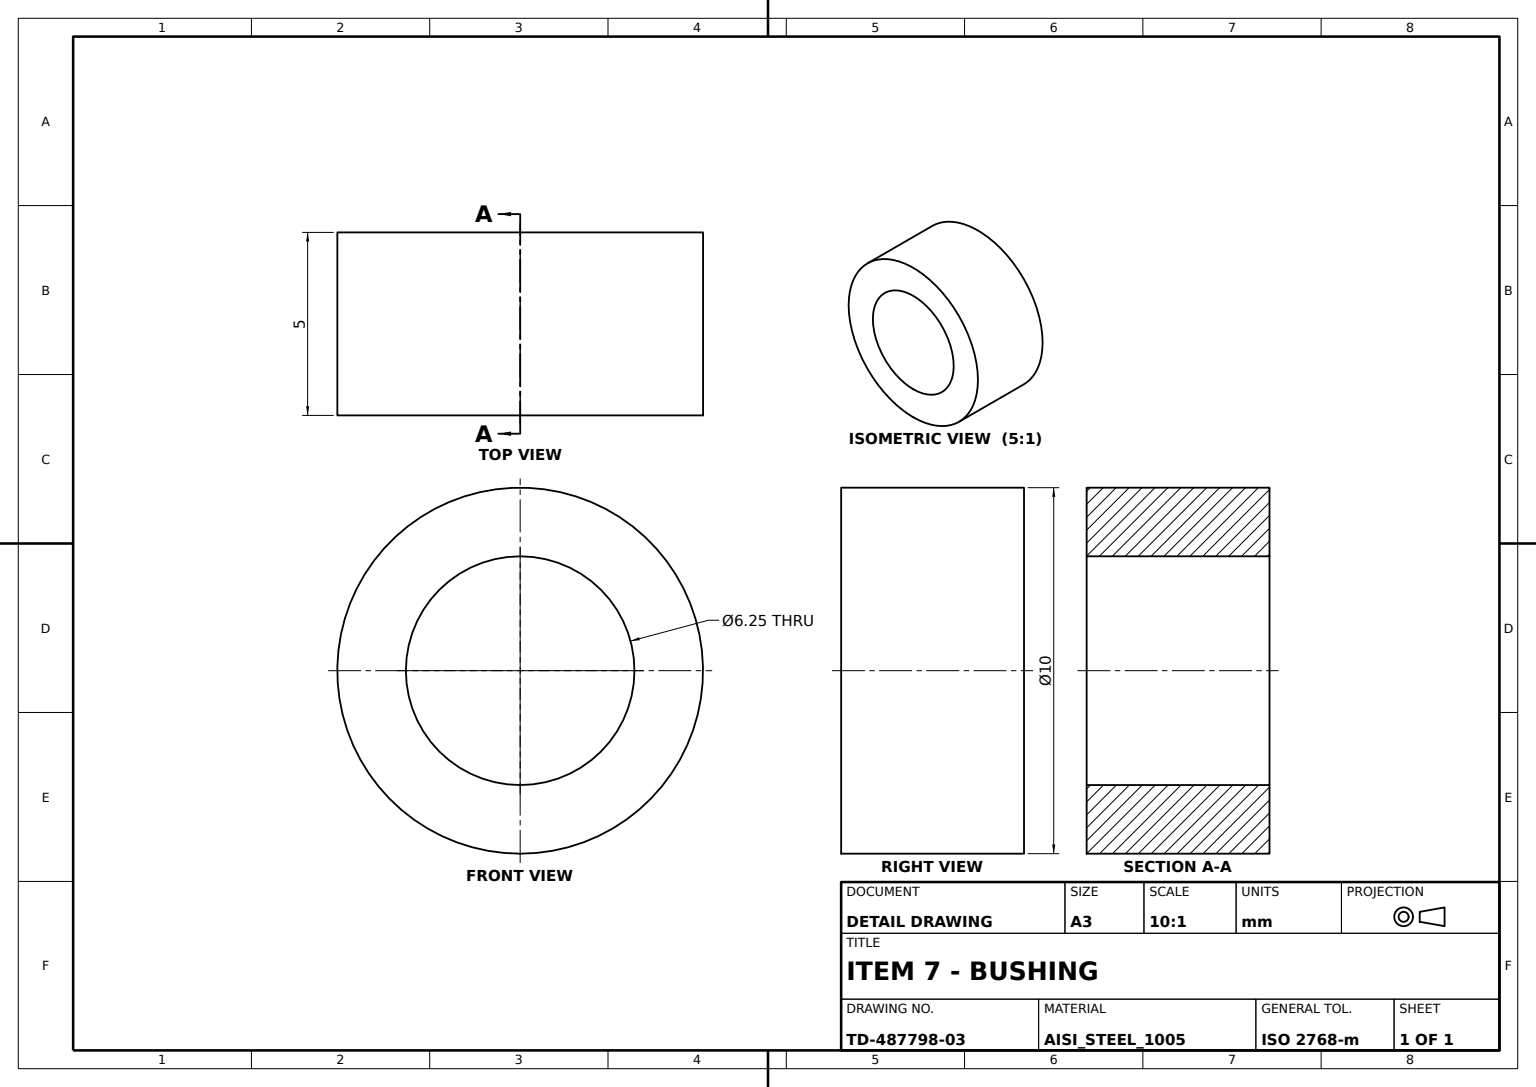
ISO-10303-21;
HEADER;
FILE_DESCRIPTION((''),'2;1');
FILE_NAME('','',(''),(''),'','','');
FILE_SCHEMA(('AUTOMOTIVE_DESIGN'));
ENDSEC;
DATA;
#1=APPLICATION_CONTEXT('');
#2=PRODUCT_CONTEXT('',#1,'mechanical');
#3=PRODUCT('','','',(#2));
#4=PRODUCT_DEFINITION_FORMATION('','',#3);
#5=PRODUCT_DEFINITION_CONTEXT('',#1,'design');
#6=PRODUCT_DEFINITION('','',#4,#5);
#7=PRODUCT_DEFINITION_SHAPE('','',#6);
#8=(LENGTH_UNIT()NAMED_UNIT(*)SI_UNIT(.MILLI.,.METRE.));
#9=(NAMED_UNIT(*)PLANE_ANGLE_UNIT()SI_UNIT($,.RADIAN.));
#10=(NAMED_UNIT(*)SI_UNIT($,.STERADIAN.)SOLID_ANGLE_UNIT());
#11=UNCERTAINTY_MEASURE_WITH_UNIT(LENGTH_MEASURE(0.005),#8,'distance_accuracy_value','');
#12=(GEOMETRIC_REPRESENTATION_CONTEXT(3)GLOBAL_UNCERTAINTY_ASSIGNED_CONTEXT((#11))GLOBAL_UNIT_ASSIGNED_CONTEXT((#8,#9,#10))REPRESENTATION_CONTEXT('',''));
#13=CARTESIAN_POINT('',(5.,0.,5.));
#14=VERTEX_POINT('',#13);
#15=CARTESIAN_POINT('',(0.,0.,5.));
#16=DIRECTION('',(0.,0.,1.));
#17=DIRECTION('',(1.,0.,0.));
#18=AXIS2_PLACEMENT_3D('',#15,#16,#17);
#19=CIRCLE('',#18,5.);
#20=EDGE_CURVE('',#14,#14,#19,.T.);
#21=ORIENTED_EDGE('',*,*,#20,.F.);
#22=EDGE_LOOP('',(#21));
#23=FACE_BOUND('',#22,.T.);
#24=CARTESIAN_POINT('',(5.,0.,0.));
#25=VERTEX_POINT('',#24);
#26=CARTESIAN_POINT('',(0.,0.,0.));
#27=AXIS2_PLACEMENT_3D('',#26,#16,#17);
#28=CIRCLE('',#27,5.);
#29=EDGE_CURVE('',#25,#25,#28,.T.);
#30=ORIENTED_EDGE('',*,*,#29,.T.);
#31=EDGE_LOOP('',(#30));
#32=FACE_BOUND('',#31,.T.);
#33=DIRECTION('',(0.,0.,-1.));
#34=DIRECTION('',(-1.,0.,0.));
#35=AXIS2_PLACEMENT_3D('',#15,#33,#34);
#36=CYLINDRICAL_SURFACE('',#35,5.);
#37=ADVANCED_FACE('',(#23,#32),#36,.T.);
#38=CARTESIAN_POINT('',(3.125,0.,5.));
#39=VERTEX_POINT('',#38);
#40=CIRCLE('',#18,3.125);
#41=EDGE_CURVE('',#39,#39,#40,.T.);
#42=ORIENTED_EDGE('',*,*,#41,.T.);
#43=EDGE_LOOP('',(#42));
#44=FACE_BOUND('',#43,.T.);
#45=CARTESIAN_POINT('',(3.125,0.,0.));
#46=VERTEX_POINT('',#45);
#47=CIRCLE('',#27,3.125);
#48=EDGE_CURVE('',#46,#46,#47,.T.);
#49=ORIENTED_EDGE('',*,*,#48,.F.);
#50=EDGE_LOOP('',(#49));
#51=FACE_BOUND('',#50,.T.);
#52=CYLINDRICAL_SURFACE('',#35,3.125);
#53=ADVANCED_FACE('',(#44,#51),#52,.F.);
#54=ORIENTED_EDGE('',*,*,#20,.T.);
#55=EDGE_LOOP('',(#54));
#56=FACE_BOUND('',#55,.T.);
#57=ORIENTED_EDGE('',*,*,#41,.F.);
#58=EDGE_LOOP('',(#57));
#59=FACE_BOUND('',#58,.T.);
#60=PLANE('',#18);
#61=ADVANCED_FACE('',(#56,#59),#60,.T.);
#62=ORIENTED_EDGE('',*,*,#29,.F.);
#63=EDGE_LOOP('',(#62));
#64=FACE_BOUND('',#63,.T.);
#65=ORIENTED_EDGE('',*,*,#48,.T.);
#66=EDGE_LOOP('',(#65));
#67=FACE_BOUND('',#66,.T.);
#68=PLANE('',#27);
#69=ADVANCED_FACE('',(#64,#67),#68,.F.);
#70=CLOSED_SHELL('',(#37,#53,#61,#69));
#71=MANIFOLD_SOLID_BREP('',#70);
#72=ADVANCED_BREP_SHAPE_REPRESENTATION('',(#71),#12);
#73=SHAPE_DEFINITION_REPRESENTATION(#7,#72);
ENDSEC;
END-ISO-10303-21;
